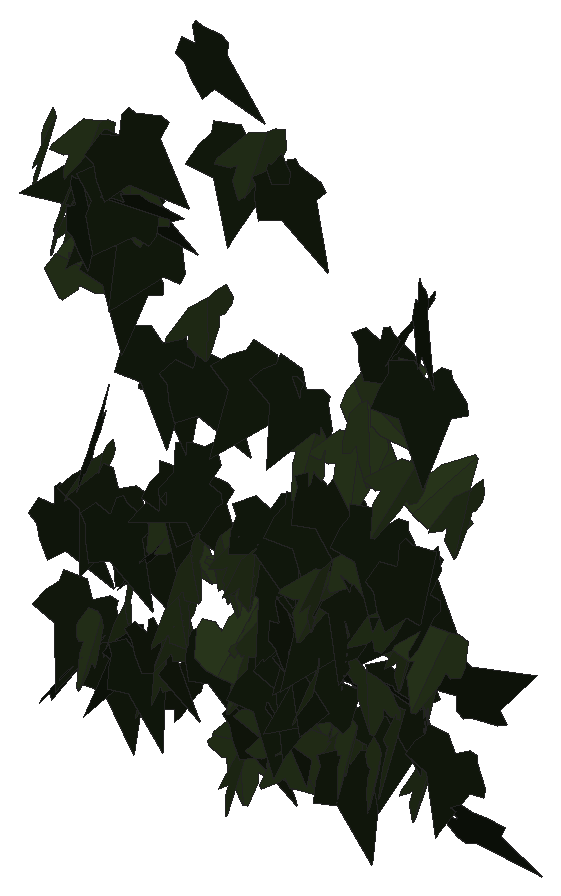
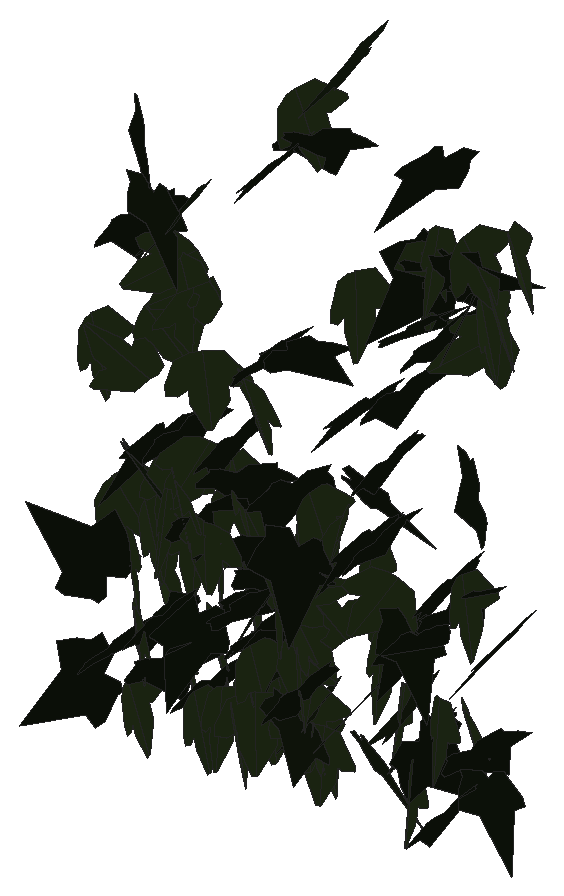
# SketchUp Ruby script. Lengths in inches.
U = 1.inch
M = Sketchup.active_model
def pt(a) = Geom::Point3d.new(a.map { |v| v * U })
def face(e, loops, mat)
  f = e.add_face(loops[0].map { |a| pt(a) })
  loops[1..].each { |l| e.add_face(l.map { |a| pt(a) }).erase! }
  f.material = f.back_material = mat if mat
  f
end
# faces: each face lists its corners as indices into pts; further lists are holes
def faces(e, pts, list, mat = nil) = list.each { |f| face(e, (f[0].is_a?(Array) ? f : [f]).map { |l| l.map { |i| pts[i] } }, mat) }
# xy, xz, yz: faces in a plane at the given z, y or x. An outline is a flat list of corners, or four numbers for a rectangle; further outlines are holes
def ring(l) = l.size == 4 ? [[l[0], l[1]], [l[2], l[1]], [l[2], l[3]], [l[0], l[3]]] : l.each_slice(2).to_a
def flat(e, list, mat, &to3) = list.each { |f| face(e, (f[0].is_a?(Array) ? f : [f]).map { |l| ring(l).map { |u, v| to3.(u, v) } }, mat) }
def xy(e, z, list, mat = nil) = flat(e, list, mat) { |x, y| [x, y, z] }
def xz(e, y, list, mat = nil) = flat(e, list, mat) { |x, z| [x, y, z] }
def yz(e, x, list, mat = nil) = flat(e, list, mat) { |y, z| [x, y, z] }
def lines(e, pts, list) = list.each { |a, b| e.add_line(pt(pts[a]), pt(pts[b])) }
# prism: a flat outline (further loops are holes) pulled along v
def prism(e, loops, v, mat = nil)
  f = face(e, loops, mat); d = Geom::Vector3d.new(v.map { |x| x * U })
  f.pushpull(f.normal.samedirection?(d) ? d.length : -d.length)
end
def box(e, o, s, mat = nil) = prism(e, [[o, [o[0] + s[0], o[1], o[2]], [o[0] + s[0], o[1] + s[1], o[2]], [o[0], o[1] + s[1], o[2]]]], [0, 0, s[2]], mat)
def at(x, y, z, deg = 0) = Geom::Transformation.translation(pt([x, y, z])) * Geom::Transformation.rotation(ORIGIN, Z_AXIS, deg.degrees)
def axes(o, x, y, z) = Geom::Transformation.new([*x, 0, *y, 0, *z, 0, *pt(o).to_a, 1])
def part(name) = M.definitions.add(name)
# library, detail: a bought-in or finely detailed component or shape, given as its bounding box
def library(name, o, s) = part(name).tap { |d| box(d.entities, o, s) }
def detail(e, o, s) = box(e.add_group.entities, o, s)
def put(e, d, t, mat = nil) = e.add_instance(d, t).tap { |i| i.material = mat if mat }
def group(e, t, mat = nil) = e.add_group.tap { |g| g.transformation = t; g.material = mat if mat }.entities
root = M.entities
M.materials.add("efeu1").color = [18, 25, 13]
M.materials.add("efeu2").color = [43, 57, 29]
c1 = part("ivyleaf_9")
p = [[1.54,2.16,1.25],[1.36,2.04,1.19],[-0.21,0.99,0.68],[-0.71,1.11,0.82],[-0.85,0.86,0.67],[-0.8,0.17,0.21],
  [-0.9,-0.01,0.1],[-0.67,-0.16,-0.02],[-0.08,-0.08,-0.05],[-0.03,-0.6,-0.4],[0.65,-0.88,-0.66],[0.83,-0.6,-0.49],
  [1.29,-0.42,-0.43],[1.8125,-0.07,-0.26],[1.21,0.44,0.15]]
faces(c1.entities,p,[[0,1,2,3,4,5,6,7,8,9,10,11,12,13,14]],"efeu1")
c2 = part("ivyleaf_10")
p = [[0,0.5,-0.03],[-0.0625,2.02,-0.43],[-0.19,2.01,-0.46],[-0.54,1.05,-0.29],[-0.52,0.625,-0.18],[-0.83,0.76,-0.28],
  [-1.16,0.64,-0.33],[-1.15,0.33,-0.24],[-0.77,-0.39,0.02],[-0.3,-0.51,0.16],[0.04,-0.48,0.23],[-0.02,2.01,-0.4375],
  [-0.06,2.01,-0.43],[0.04,-0.49,0.23],[0.67,-0.49,0.14],[1.38,0.36,-0.2],[1.375,0.51,-0.24],[0.81,0.65,-0.19],
  [0.62,0.59,-0.15],[0.6,1.09,-0.28],[0.5,1.23,-0.31]]
faces(c2.entities,p,[[0,1,2,3,4,5,6,7,8,9,10],[11,12,0,13,14,15,16,17,18,19,20]],"efeu2")
put(root,c1,axes([565.9,123.85,299.61],[0.34552,-0.66975,-0.96332],[-0.10603,0.98229,-0.72097],[1.16846,0.28718,0.21944]))
put(root,c1,axes([564.69,123.4,286.58],[0.10354,0.28094,1.16639],[-0.02871,1.17097,-0.27949],[-1.1994,-0.00378,0.10738]))
put(root,c2,axes([573.9,124.27,280.92],[0.39071,-1.01895,-0.39398],[-0.14311,0.36707,-1.09129],[1.08305,0.41609,-0.00207]))
put(root,c2,axes([577.47,125.01,289.85],[-0.20602,-0.98037,0.64481],[-0.05146,-0.64649,-0.99937],[1.17228,-0.20068,0.06945]))
put(root,c2,axes([576.94,125.07,279.81],[0.56239,-0.82353,0.69398],[0.41009,-0.56017,-0.99706],[0.99581,0.69578,0.01867]))
put(root,c1,axes([577.93,125.125,296.59],[0.05837,-0.28146,-1.20012],[1.21647,-0.18103,0.10162],[-0.19923,-1.18782,0.26888]))
put(root,c1,axes([573.21,125.41,280.35],[-0.18922,-0.91859,0.6675],[0.21671,-0.69348,-0.89292],[1.11464,-0.02111,0.28691]))
put(root,c2,axes([576.38,124.38,281.65],[-1.12257,0.22492,0.28231],[-0.28618,0.00746,-1.14389],[-0.21998,-1.1575,0.04749]))
put(root,c2,axes([569.04,124.52,293.74],[-0.22402,-1.19245,-0.19776],[0.03769,0.19414,-1.21331],[1.20815,-0.22717,0.00118]))
put(root,c1,axes([564.8,124.68,283.91],[0.46556,-1.0279,-0.3823],[-0.08313,0.38105,-1.12578],[1.09354,0.46659,0.07718]))
put(root,c1,axes([578.2,125.09,293.74],[-0.16971,-1.21507,-0.17882],[0.0002,0.18049,-1.22662],[1.22815,-0.16794,-0.02451]))
put(root,c2,axes([561.83,124.85,298.03],[0.61646,-1.04031,0.07335],[0.03084,-0.06699,-1.20922],[1.04244,0.61718,-0.0076]))
put(root,c1,axes([563.77,124.07,296.08],[0.69051,-0.30849,-0.95222],[-0.73274,0.63231,-0.7362],[0.6819,0.99183,0.17317]))
put(root,c2,axes([570.54,124.91,284.78],[-0.03529,-1.1537,0.20714],[-0.01912,-0.20664,-1.15417],[1.17199,-0.03811,-0.01259]))
put(root,c2,axes([573.87,125.05,284.35],[-0.35024,-1.02209,0.44967],[-0.11916,-0.43437,-1.08012],[1.11026,-0.36904,0.02593]))
put(root,c2,axes([568.4,124.42,283.625],[0.20702,-1.06992,-0.47692],[0.08135,0.49627,-1.07802],[1.16857,0.155,0.15953]))
put(root,c2,axes([573.98,124.81,284.9],[0.38958,-1.14716,-0.05399],[-0.0176,0.05104,-1.21151],[1.14829,0.38998,-0.00026]))
put(root,c1,axes([573.87,125.59,280.21],[-0.72856,-0.6525,0.6229],[-0.21971,-0.64821,-0.936],[0.87492,-0.70613,0.28364]))
put(root,c2,axes([563.33,124.34,293.74],[-0.59715,-0.30203,-1.00849],[0.93255,0.38625,-0.66786],[0.48851,-1.10655,0.04215]))
put(root,c2,axes([574.93,125,278.58],[0.81015,-0.83197,0.13658],[0.10403,-0.08932,-1.16119],[0.83666,0.81671,0.01214]))
put(root,c1,axes([566.53,125.26,290.98],[-0.02235,-1.20348,-0.10073],[0.02251,0.10032,-1.20351],[1.20748,-0.02415,0.02057]))
put(root,c2,axes([567.75,124.5625,281.62],[0.11814,-1.09145,-0.44038],[0.08469,0.44932,-1.09091],[1.17389,0.07742,0.12302]))
put(root,c2,axes([570.86,124.78,284.4],[0.14735,-1.16182,-0.19247],[0.03453,0.19815,-1.16967],[1.17715,0.13962,0.05841]))
put(root,c1,axes([571.84,125.3,279.72],[-0.43071,-1.05196,-0.21086],[0.16971,0.15756,-1.13268],[1.05938,-0.45294,0.09573]))
put(root,c1,axes([568.66,124.98,286.49],[-1.11497,0.25235,0.30009],[-0.29222,0.06832,-1.14317],[-0.26143,-1.15263,-0.00206]))
put(root,c2,axes([570.95,125.16,300.57],[-0.27202,-1.16742,0.29223],[-0.00002,-0.2996,-1.19687],[1.20344,-0.26389,0.06603]))
put(root,c2,axes([563.65,125.07,278.93],[0.88162,-0.72881,0.01205],[0.005,-0.01287,-1.14385],[0.7289,0.88161,-0.00673]))
put(root,c1,axes([564.76,125.54,293.8],[-0.02639,-1.19226,0.13828],[0.01776,-0.13868,-1.19238],[1.20012,-0.02416,0.02069]))
put(root,c2,axes([569.75,124.77,284.29],[-0.24137,1.13588,-0.00602],[0.00661,-0.00475,-1.16123],[-1.13588,-0.2414,-0.00548]))
put(root,c1,axes([565.17,125.48,296.49],[-1.09708,-0.48625,0.11292],[-0.11852,-0.01113,-1.19941],[0.48492,-1.10282,-0.03768]))
put(root,c2,axes([562.44,125.15,295.73],[0.67083,-1.02597,0.04185],[0.01483,-0.0403,-1.22578],[1.02672,0.67092,-0.00964]))
put(root,c2,axes([570.1,125.17,276.26],[0.41999,-1.10899,0.09128],[0.03305,-0.08509,-1.18585],[1.11225,0.42129,0.00077]))
put(root,c2,axes([572.82,124.71,277.48],[-0.43544,-0.94744,-0.49277],[0.24664,0.42855,-1.04192],[1.03906,-0.49877,0.04081]))
put(root,c1,axes([571.02,125.7,291.14],[-0.91463,-0.73767,0.16139],[-0.09121,-0.14371,-1.17379],[0.74959,-0.91758,0.05409]))
put(root,c1,axes([571.9,125.69,277.97],[0.2464,-0.86973,0.69875],[0.31587,-0.63192,-0.89794],[1.07,0.38683,0.10417]))
put(root,c1,axes([576.22,125.21,294.5],[0.62668,-1.05488,-0.11701],[0.03806,0.15814,-1.22177],[1.06066,0.61758,0.11298]))
put(root,c1,axes([570,125.66,299.9],[-0.68474,-0.95309,-0.27578],[0.31025,0.1126,-1.15947],[0.94244,-0.72955,0.18133]))
put(root,c2,axes([576.71,124.98,284.11],[-0.45378,-1.04343,-0.31555],[0.09365,0.30321,-1.13733],[1.08607,-0.46211,-0.03377]))
put(root,c2,axes([569.79,124.61,280.18],[0.67973,0.71896,-0.67941],[0.4754,0.48548,0.98936],[0.86746,-0.82942,-0.00983]))
put(root,c2,axes([578.41,125.73,283.16],[-0.48278,-0.92583,0.60935],[0.0442,-0.6802,-0.99846],[1.10748,-0.37644,0.30548]))
put(root,c2,axes([570.31,125.85,280.63],[0.30439,-0.91835,0.667],[0.26452,-0.61416,-0.96631],[1.10376,0.40045,0.04764]))
put(root,c1,axes([572.23,126.04,279.92],[-0.23903,-1.11984,0.32087],[0.02511,-0.33243,-1.14148],[1.16463,-0.22267,0.09047]))
put(root,c2,axes([562.76,125.34,295.39],[0.37749,-1.14486,-0.10282],[-0.00403,0.1069,-1.20513],[1.14946,0.37635,0.02954]))
put(root,c2,axes([575.9,125.22,277.875],[0.70945,-0.86339,-0.28129],[-0.09332,0.28575,-1.11244],[0.90325,0.70766,0.106]))
put(root,c1,axes([568.33,125.02,303.58],[0.88786,-0.7157,-0.48462],[-0.18987,0.51628,-1.11031],[0.84323,0.86983,0.26026]))
put(root,c2,axes([575.64,125.24,291.41],[0.25081,1.16247,-0.08142],[-0.10562,-0.06027,-1.18578],[-1.16052,0.25672,0.09032]))
put(root,c1,axes([567.06,125.99,285.21],[-0.02312,-1.1499,0.25377],[0.02504,-0.25424,-1.14975],[1.1773,-0.01718,0.02944]))
put(root,c1,axes([564.22,125.91,296.6],[-0.86005,-0.17057,0.82517],[-0.7849,-0.26669,-0.8732],[0.30648,-1.16166,0.07931]))
put(root,c2,axes([563.03,125.81,297.89],[-0.16776,-1.10569,0.46803],[0.06215,-0.47994,-1.11155],[1.19906,-0.12982,0.12309]))
put(root,c1,axes([571.9375,126.25,290.71],[-0.35897,-1.02949,0.48739],[0.00413,-0.51219,-1.07884],[1.13902,-0.32259,0.15751]))
put(root,c2,axes([574.62,125.12,282.26],[0.68638,-0.78997,-0.53731],[-0.16766,0.55173,-1.02535],[0.94055,0.67483,0.20933]))
put(root,c1,axes([565.16,125.6875,278.11],[0.31545,-1.09083,-0.13741],[-0.01476,0.13874,-1.13527],[1.09935,0.31487,0.02419]))
put(root,c1,axes([573.5625,126.2,282.65],[-0.7771,-0.87318,0.27668],[-0.08331,-0.29396,-1.16169],[0.91217,-0.77073,0.12961]))
put(root,c1,axes([574.49,125.68,277.04],[0.15518,-1.10249,-0.27068],[-0.00803,0.27212,-1.11297],[1.1352,0.15263,0.02913]))
put(root,c2,axes([565.25,125.32,296.58],[-1.18841,0.01105,0.20206],[-0.20235,-0.0512,-1.18731],[-0.0023,-1.20438,0.05232]))
put(root,c1,axes([575.58,126.02,286.61],[-0.15128,-1.19334,0.00205],[-0.02262,0.0008,-1.20268],[1.19313,-0.15129,-0.02254]))
put(root,c2,axes([567.42,125.14,280.51],[0.12158,-1.0763,-0.59242],[-0.03405,0.59213,-1.08277],[1.2281,0.12297,0.02863]))
put(root,c1,axes([561.86,125.3,283.01],[0.67697,-0.82498,-0.51444],[-0.1363,0.54014,-1.04556],[0.96264,0.65665,0.21374]))
put(root,c1,axes([571.01,125.625,285.88],[-0.00092,-1.05831,-0.50356],[-0.00267,0.50356,-1.05831],[1.172,0.00032,-0.00281]))
put(root,c2,axes([570.36,126.18,279.91],[-0.09089,-0.84923,0.82594],[0.03477,-0.82992,-0.8495],[1.18413,-0.04081,0.08834]))
put(root,c1,axes([563.66,126.27,283.875],[-0.45654,-1.04318,0.27442],[0.02791,-0.30932,-1.12939],[1.07831,-0.43366,0.14542]))
put(root,c2,axes([575.31,125.34,292.08],[0.63435,0.07075,1.00459],[0.94408,0.37156,-0.62231],[-0.35061,1.12852,0.14192]))
put(root,c1,axes([565.72,125.58,279.1875],[0.7189,-0.87906,-0.16659],[-0.00994,0.20585,-1.12909],[0.89465,0.70866,0.12132]))
put(root,c1,axes([571.89,125.15,281.96],[0.81616,-0.47565,-0.74425],[-0.53668,0.53778,-0.93222],[0.70152,0.96479,0.1527]))
put(root,c1,axes([569.99,125.59,277.43],[0.73037,-0.87128,-0.24651],[-0.07353,0.2586,-1.13184],[0.90249,0.72618,0.10729]))
put(root,c1,axes([565.25,126.48,294.37],[-0.59455,-0.94767,0.40441],[0.0622,-0.49907,-1.07804],[1.02847,-0.51766,0.29898]))
put(root,c2,axes([571.8,125.625,277.35],[-0.61476,-0.98924,-0.02006],[0.01546,0.01401,-1.16468],[0.98932,-0.61492,0.00574]))
put(root,c1,axes([567.75,125.56,290.3125],[0.49491,-0.96743,-0.49733],[0.05731,0.56881,-1.04946],[1.08626,0.41076,0.28196]))
put(root,c2,axes([569.78,125.61,276.23],[-1.13963,-0.0376,0.07781],[-0.07205,-0.15481,-1.13008],[0.04772,-1.13175,0.15199]))
put(root,c2,axes([566.44,125.27,278.88],[0.48177,-0.88599,-0.61923],[0.01017,0.68163,-0.96737],[1.08089,0.38849,0.2851]))
put(root,c2,axes([570.46,125.73,277.5],[-0.64762,-0.9441,0.09396],[-0.05907,-0.07342,-1.14485],[0.94692,-0.65027,-0.00715]))
put(root,c2,axes([576.04,125.47,292.97],[-0.72409,-0.18698,-0.966],[0.96075,0.12448,-0.74424],[0.21234,-1.20082,0.07327]))
put(root,c1,axes([576.87,125.39,285.82],[0.53362,-0.82192,-0.80551],[-0.18059,0.81709,-0.95336],[1.13657,0.51572,0.22671]))
put(root,c1,axes([565.13,125.14,296.19],[1.15489,0.34027,0.01562],[-0.01215,0.09635,-1.20015],[-0.34041,1.15097,0.09585]))
put(root,c1,axes([562.62,125.35,277.0625],[-0.32773,1.08765,-0.05036],[-0.02087,-0.05886,-1.13536],[-1.08862,-0.32631,0.03693]))
put(root,c1,axes([574.41,126.37,283.81],[-0.4094,-1.11067,0.00526],[-0.00091,-0.00527,-1.18373],[1.11069,-0.4094,0.00096]))
put(root,c2,axes([575.1,125.54,285.54],[-0.74741,-0.70583,-0.57898],[0.53334,0.2697,-1.01727],[0.74092,-0.90615,0.14822]))
put(root,c2,axes([579.32,125.92,289.14],[-0.00014,-1.20744,0.01009],[-0.00031,-0.01009,-1.20744],[1.20749,-0.00014,-0.00031]))
put(root,c2,axes([572.49,125.94,289.16],[1.06855,-0.54273,-0.06312],[-0.056,0.02912,-1.19848],[0.54351,1.07002,0.00061]))
put(root,c1,axes([562.34,126.51,278.94],[-0.4719,-1.03697,0.14446],[-0.03921,-0.14084,-1.13907],[1.04625,-0.47299,0.02247]))
put(root,c1,axes([577.55,125.97,284.75],[-1.3301,0.61092,-0.11745],[0.10552,-0.05166,-1.46369],[-0.61309,-1.33428,0.00289]))
put(root,c1,axes([572.75,126.35,286.06],[-0.55373,-1.01419,-0.31515],[0.30167,0.19057,-1.14333],[1.01828,-0.60796,0.16734]))
put(root,c1,axes([573.11,126.15,287.28],[0.24156,-1.15797,-0.22132],[-0.03889,0.21797,-1.18288],[1.17829,0.24459,0.00633]))
put(root,c2,axes([574.52,126.11,289.46],[-0.97948,-0.65909,0.17702],[0.01424,-0.32933,-1.14737],[0.6823,-0.93929,0.27807]))
put(root,c1,axes([564.7,126.43,278.33],[-0.29876,0.50255,-0.98464],[0.30983,-0.94102,-0.57429],[-1.06116,-0.41623,0.10954]))
put(root,c2,axes([572.14,126.21,278.81],[-0.0945,-1.17257,0.14511],[0.01021,-0.14638,-1.17617],[1.18147,-0.09253,0.02177]))
put(root,c1,axes([571.16,126.14,298.84],[0.46173,-1.07055,-0.28617],[0.07728,0.34037,-1.14863],[1.10544,0.42337,0.19983]))
put(root,c1,axes([567.42,125.86,285.3],[0.49982,-0.86949,-0.61124],[-0.10753,0.63063,-0.98499],[1.05739,0.47513,0.18877]))
put(root,c2,axes([576.72,126.21,282.88],[0.28112,-1.1435,-0.00813],[-0.00012,0.00834,-1.17754],[1.14352,0.28112,0.00188]))
put(root,c1,axes([571.31,126.72,282.93],[-0.75385,-0.89375,-0.0152],[0.05376,-0.02549,-1.16781],[0.89226,-0.75358,0.05753]))
put(root,c1,axes([577.06,125.61,295.09],[-0.45513,1.10166,0.24911],[-0.0867,0.23371,-1.19194],[-1.12614,-0.46323,-0.00892]))
put(root,c2,axes([566.51,126.07,283.55],[-0.93989,-0.3132,-0.59798],[0.62273,-0.00665,-0.97531],[0.26054,-1.11396,0.17395]))
put(root,c2,axes([562.95,126.1875,284.76],[0.08144,-1.17825,-0.16844],[-0.01866,0.16755,-1.18104],[1.19008,0.08325,-0.00699]))
put(root,c1,axes([572.36,127.12,281.19],[-0.59197,-0.84479,0.49042],[-0.13923,-0.49462,-1.02009],[0.96685,-0.58846,0.15337]))
put(root,c2,axes([575.18,126.49,284.46],[0.95044,-0.68938,0.15691],[0.16491,-0.03949,-1.17237],[0.68751,0.9625,0.06429]))
put(root,c2,axes([564.36,125.94,297.77],[0.10858,-1.02035,-0.63494],[0.03743,0.64009,-1.02222],[1.20119,0.07229,0.08924]))
put(root,c1,axes([565.61,125.93,282.31],[-0.26543,1.1221,-0.04837],[0.01816,-0.04541,-1.15305],[-1.123,-0.26595,-0.00721]))
put(root,c2,axes([570.06,126.26,279.55],[0.4379,-1.02538,-0.32714],[-0.03286,0.34027,-1.11054],[1.0758,0.42777,0.09924]))
put(root,c2,axes([570.12,126.9,282.47],[0.21123,0.29077,1.11553],[-0.81625,-0.76313,0.35348],[0.81406,-0.84063,0.06497]))
put(root,c1,axes([564.91,126.46,282.42],[0.22197,-0.98217,-0.60833],[-0.06494,0.60787,-1.00512],[1.15347,0.22322,0.06048]))
put(root,c2,axes([564.13,126.1,279.49],[0.20802,-0.92707,-0.71091],[-0.12522,0.70024,-0.9498],[1.16154,0.24152,0.02493]))
put(root,c2,axes([577.41,126.13,288.4],[0.78491,0.28257,-0.86056],[0.81171,0.28582,0.83421],[0.4019,-1.12913,-0.00419]))
put(root,c1,axes([577.68,127.32,277.93],[-0.17762,-1.06405,0.36521],[0.08657,-0.38156,-1.0696],[1.12164,-0.13905,0.14039]))
put(root,c1,axes([565.74,127.01,289.33],[0.19454,-1.15045,-0.03245],[-0.00317,0.03238,-1.16678],[1.15091,0.19456,0.00228]))
put(root,c2,axes([577.5,126.37,281.5625],[0.66586,-0.76445,-0.64907],[-0.31594,0.57953,-1.00667],[0.95177,0.72719,0.11993]))
put(root,c1,axes([567.38,126.87,278.83],[0.51306,-1.04605,-0.1518],[0.02621,0.18128,-1.16058],[1.05668,0.5034,0.10249]))
put(root,c2,axes([571.75,126.78,277.34],[-0.94847,-0.68999,0.0723],[0.00903,-0.13474,-1.16733],[0.6937,-0.94163,0.11406]))
put(root,c2,axes([573.83,126.75,283.47],[1.17196,-0.01511,0.0935],[0.0947,0.16889,-1.15972],[0.00147,1.16349,0.16955]))
put(root,c1,axes([566.8125,126.75,277.57],[-0.90758,0.67082,0.127],[-0.09721,0.08215,-1.12856],[-0.67578,-0.91274,-0.00823]))
put(root,c1,axes([578.72,126.48,276.11],[1.13568,0.05518,0.26359],[0.26352,0.00784,-1.13701],[-0.05552,1.16584,-0.00483]))
put(root,c1,axes([562.98,127.32,276.61],[0.18491,-1.14119,-0.0532],[0.02526,0.05796,-1.15557],[1.14215,0.18347,0.03417]))
put(root,c2,axes([572.35,126.97,276.86],[0.53499,-1.03638,-0.20639],[-0.04576,0.2084,-1.16506],[1.05574,0.53421,0.05409]))
put(root,c2,axes([570.6,126.8,282.41],[-0.83975,0.78211,0.26976],[-0.34799,0.01481,-1.1262],[-0.75058,-0.88189,0.22033]))
put(root,c1,axes([569.27,127.42,279.28],[0.13068,-1.1403,-0.10433],[-0.02127,0.10258,-1.14773],[1.14487,0.13207,-0.00941]))
put(root,c1,axes([570.22,126.22,277.16],[0.04455,0.9438,0.64907],[-0.26351,0.64059,-0.91338],[-1.11473,-0.11371,0.24185]))
put(root,c1,axes([575.08,127.5625,278.46],[-0.48206,-1.03443,-0.13023],[0.04676,0.12188,-1.1412],[1.04155,-0.48424,-0.00904]))
put(root,c1,axes([578.14,127.07,280.63],[0.09,-0.19273,1.21554],[1.15448,-0.40909,-0.15035],[0.42645,1.14816,0.15047]))
put(root,c1,axes([575.23,127.4,280.06],[0.19754,-1.11497,-0.23156],[-0.0095,0.2334,-1.13192],[1.13873,0.19537,0.03073]))
put(root,c2,axes([575.49,126.84,283.99],[0.29932,-1.00342,-0.53711],[0.06711,0.56997,-1.0274],[1.13615,0.23068,0.20219]))
put(root,c2,axes([573.01,126.94,277.2],[-0.05961,-1.05176,-0.41149],[0.0244,0.41077,-1.05345],[1.12913,-0.0644,0.00104]))
put(root,c2,axes([564.75,126.75,277.07],[0.31729,-0.83678,-0.7553],[-0.10986,0.75796,-0.88588],[1.12188,0.31088,0.12687]))
put(root,c1,axes([574.32,126.68,280],[0.90637,0.56279,-0.46541],[-0.53373,0.00415,-1.03439],[-0.49847,1.01887,0.26129]))
put(root,c1,axes([569.76,126.89,284.33],[0.15355,1.16271,-0.02225],[0.01836,-0.02487,-1.17261],[-1.16278,0.15315,-0.02146]))
put(root,c2,axes([576.22,127.51,279.57],[0.78498,-0.84041,-0.06617],[0.07547,0.16011,-1.13821],[0.83963,0.77132,0.16417]))
put(root,c2,axes([573.44,127.67,277.18],[0.08714,-1.14167,-0.01643],[-0.00156,0.01636,-1.14499],[1.14179,0.08715,-0.00031]))
put(root,c2,axes([576.15,127.83,276.82],[0.23059,-1.1117,0.0903],[0.00813,-0.09053,-1.13531],[1.11533,0.2305,-0.0104]))
